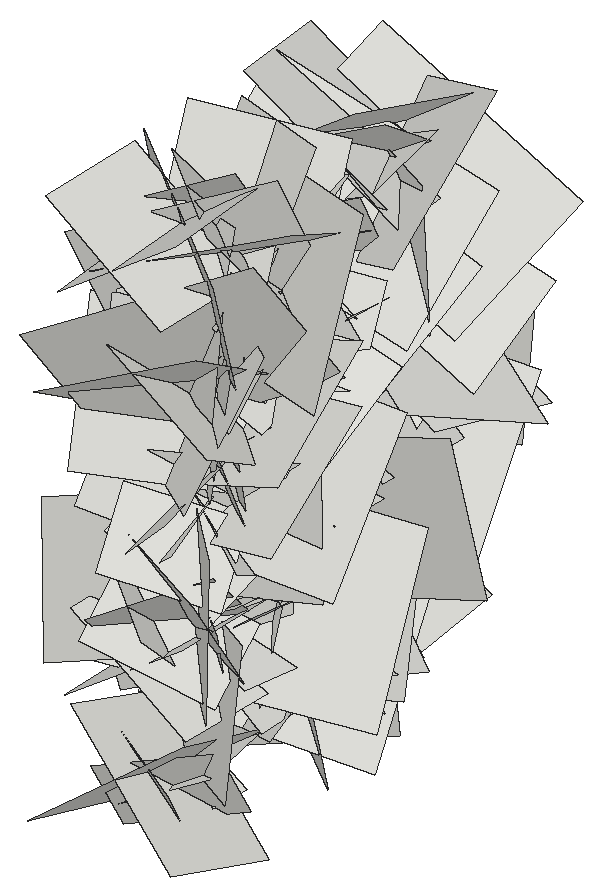
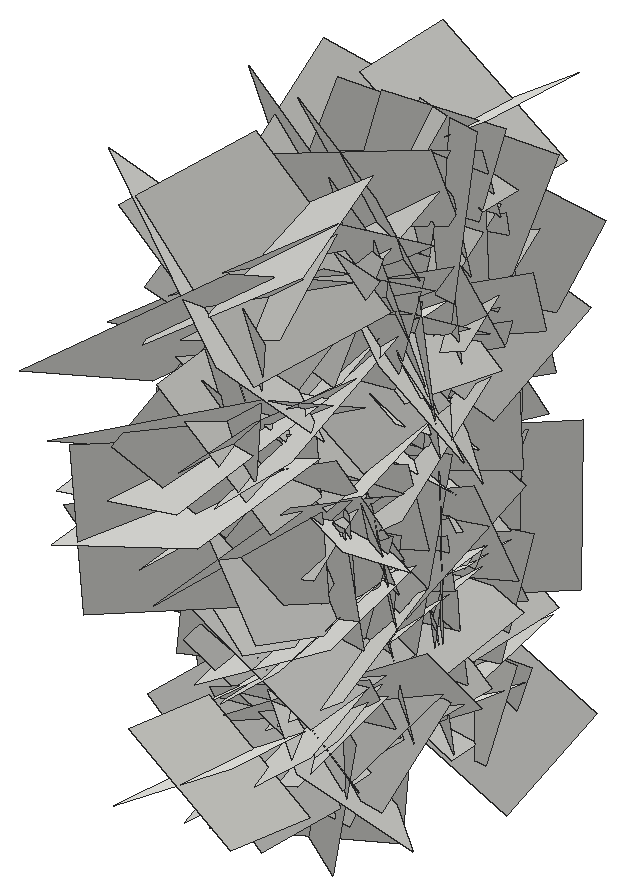
# SketchUp Ruby script. Lengths in inches.
U = 1.inch
M = Sketchup.active_model
def pt(a) = Geom::Point3d.new(a.map { |v| v * U })
def face(e, loops, mat)
  f = e.add_face(loops[0].map { |a| pt(a) })
  loops[1..].each { |l| e.add_face(l.map { |a| pt(a) }).erase! }
  f.material = f.back_material = mat if mat
  f
end
# faces: each face lists its corners as indices into pts; further lists are holes
def faces(e, pts, list, mat = nil) = list.each { |f| face(e, (f[0].is_a?(Array) ? f : [f]).map { |l| l.map { |i| pts[i] } }, mat) }
# xy, xz, yz: faces in a plane at the given z, y or x. An outline is a flat list of corners, or four numbers for a rectangle; further outlines are holes
def ring(l) = l.size == 4 ? [[l[0], l[1]], [l[2], l[1]], [l[2], l[3]], [l[0], l[3]]] : l.each_slice(2).to_a
def flat(e, list, mat, &to3) = list.each { |f| face(e, (f[0].is_a?(Array) ? f : [f]).map { |l| ring(l).map { |u, v| to3.(u, v) } }, mat) }
def xy(e, z, list, mat = nil) = flat(e, list, mat) { |x, y| [x, y, z] }
def xz(e, y, list, mat = nil) = flat(e, list, mat) { |x, z| [x, y, z] }
def yz(e, x, list, mat = nil) = flat(e, list, mat) { |y, z| [x, y, z] }
def lines(e, pts, list) = list.each { |a, b| e.add_line(pt(pts[a]), pt(pts[b])) }
# prism: a flat outline (further loops are holes) pulled along v
def prism(e, loops, v, mat = nil)
  f = face(e, loops, mat); d = Geom::Vector3d.new(v.map { |x| x * U })
  f.pushpull(f.normal.samedirection?(d) ? d.length : -d.length)
end
def box(e, o, s, mat = nil) = prism(e, [[o, [o[0] + s[0], o[1], o[2]], [o[0] + s[0], o[1] + s[1], o[2]], [o[0], o[1] + s[1], o[2]]]], [0, 0, s[2]], mat)
def at(x, y, z, deg = 0) = Geom::Transformation.translation(pt([x, y, z])) * Geom::Transformation.rotation(ORIGIN, Z_AXIS, deg.degrees)
def axes(o, x, y, z) = Geom::Transformation.new([*x, 0, *y, 0, *z, 0, *pt(o).to_a, 1])
def part(name) = M.definitions.add(name)
# library, detail: a bought-in or finely detailed component or shape, given as its bounding box
def library(name, o, s) = part(name).tap { |d| box(d.entities, o, s) }
def detail(e, o, s) = box(e.add_group.entities, o, s)
def put(e, d, t, mat = nil) = e.add_instance(d, t).tap { |i| i.material = mat if mat }
def group(e, t, mat = nil) = e.add_group.tap { |g| g.transformation = t; g.material = mat if mat }.entities
root = M.entities
c1 = part("Component\#6")
p = [[0.01,0,0],[0,3.24,4.54],[4.32,3.24,4.54],[4.33,0,0]]
faces(c1.entities,p,[[0,1,2,3]])
put(root,c1,axes([424.49,185.4,30.76],[0.02152,-0.00963,-1.2106],[0.23963,-1.18945,0.01326],[-1.26071,-0.22625,-0.01814]))
put(root,c1,axes([420.52,183.74,37.84],[0.08456,-0.37494,0.46177],[-0.03825,0.46199,0.38136],[0.62935,0.07846,-0.03886]))
put(root,c1,axes([420.52,188.62,32.29],[-0.0866,-0.74743,0.19758],[-0.06186,0.20408,0.74787],[0.81715,-0.06376,0.07755]))
put(root,c1,axes([420.52,184.65,28.76],[0.04824,-0.62434,-0.28052],[-0.09786,-0.28417,0.61748],[0.7189,0.00321,0.10288]))
put(root,c1,axes([424.49,186.48,30.64],[-0.03295,0.70699,0.47041],[-0.18441,0.45544,-0.69599],[-0.88105,-0.12176,0.12808]))
put(root,c1,axes([424.49,180.55,24.45],[-0.04702,0.95483,-0.28451],[0.08229,-0.28062,-0.95386],[-1.05288,-0.06457,-0.06184]))
put(root,c1,axes([424.49,184.8,33.37],[-0.19651,0.19461,-0.78555],[0.01158,-0.80522,-0.20206],[-0.85778,-0.05545,0.17724]))
put(root,c1,axes([424.49,181.12,36.49],[0.0887,0.85058,-0.45713],[-0.14057,-0.44437,-0.85112],[-1.01388,0.13603,0.07801]))
put(root,c1,axes([420.52,182.11,23.57],[-0.01533,0.32032,-0.55846],[0.07998,-0.55391,-0.31966],[0.67773,0.07262,0.02509]))
put(root,c1,axes([420.52,186.27,36.66],[-0.23271,0.08267,-1.0169],[-0.17131,-1.02986,-0.04883],[1.06781,-0.14721,-0.22945]))
put(root,c1,axes([420.52,181.88,29.24],[0.0732,0.47057,-0.46808],[-0.06498,-0.46407,-0.47558],[0.70054,-0.09222,0.00479]))
put(root,c1,axes([420.52,188.01,25.87],[-0.18323,0.88768,-0.1275],[-0.06793,-0.14175,-0.89995],[0.94816,0.16139,-0.08912]))
put(root,c1,axes([424.49,186.85,26],[-0.04759,0.74401,-0.43208],[-0.09551,-0.43435,-0.73856],[-0.90698,0.0067,0.10045]))
put(root,c1,axes([424.49,182.62,33.52],[0.16113,0.63843,0.91206],[0.00988,0.91976,-0.64538],[-1.18006,0.09488,0.11913]))
put(root,c1,axes([420.52,188.3,31.13],[-0.1103,-0.11339,-0.88165],[-0.13763,-0.87621,0.12802],[0.93214,-0.14279,-0.08543]))
put(root,c1,axes([424.49,182.86,27.86],[-0.00866,0.87216,-0.09866],[-0.12421,-0.09886,-0.86427],[-0.92206,0.00513,0.11735]))
put(root,c1,axes([420.52,188.48,31.6],[0.00806,0.51701,-0.38199],[0.06142,-0.38101,-0.51453],[0.67861,0.02834,0.0511]))
put(root,c1,axes([420.52,189.49,31],[-0.19159,0.03614,-0.77666],[0.1449,-0.78347,-0.06827],[0.81131,0.14846,-0.17121]))
put(root,c1,axes([424.49,186.8,27.07],[0.11611,-1.02809,0.5245],[0.14127,0.5346,1.02006],[-1.21522,-0.03608,0.16869]))
put(root,c1,axes([420.52,181.75,22.9],[0.07496,0.59984,0.04506],[0.05269,0.03939,-0.60235],[0.63545,-0.07402,0.04463]))
put(root,c1,axes([424.49,190.89,25.45],[0.07637,-0.93381,0.1535],[-0.06656,0.14888,0.93522],[-1.00091,-0.08115,-0.05048]))
put(root,c1,axes([424.49,189.24,21.76],[-0.15995,-0.688,0.38857],[0.02017,0.39231,0.70202],[-0.83731,0.14088,-0.05731]))
put(root,c1,axes([420.52,186.9,33.68],[-0.12726,-0.80704,-0.07778],[0.05104,-0.08559,0.81372],[0.85791,-0.11462,-0.05995]))
put(root,c1,axes([420.52,183.3,35.54],[0.06853,-0.0517,0.64839],[0.02911,0.65122,0.04919],[0.68886,-0.02238,-0.06659]))
put(root,c1,axes([424.49,182.91,34.72],[0.14912,-0.41506,0.98502],[0.044,0.99488,0.41329],[-1.13217,-0.016,0.1458]))
put(root,c1,axes([424.49,191.48,24.4],[0.24044,-0.84726,-0.84182],[0.11443,-0.83882,0.87332],[-1.26085,-0.2377,-0.08127]))
put(root,c1,axes([420.52,194.3125,23.26],[-0.02367,-0.75059,-0.08188],[0.02978,-0.08269,0.75031],[0.79979,-0.01914,-0.03036]))
put(root,c1,axes([424.49,189.58,22.99],[0.08755,-0.94666,0.34405],[0.04779,0.34833,0.94763],[-1.06661,-0.0621,0.0707]))
put(root,c1,axes([424.49,183.5625,38.07],[-0.03427,-0.86867,-0.02883],[0.01016,-0.0292,0.8692],[-0.92124,0.03199,0.01066]))
put(root,c1,axes([420.52,186.98,23.44],[-0.07046,0.41434,0.63319],[0.10971,0.63463,-0.40442],[0.79457,-0.05088,0.11199]))
put(root,c1,axes([424.49,186.99,20.26],[-0.04681,-0.17583,0.86867],[0.05724,0.86759,0.17835],[-0.93771,0.06173,-0.03248]))
put(root,c1,axes([420.52,182.78,23.92],[-0.06221,-0.24398,0.83625],[-0.07047,0.83695,0.23952],[0.92069,0.04758,0.07484]))
put(root,c1,axes([424.49,187.32,34.27],[-0.05201,-0.4187,0.7383],[0.02779,0.73844,0.42051],[-0.89926,0.04704,-0.0297]))
put(root,c1,axes([420.52,187.84,31.26],[0.01205,0.8882,0.30464],[-0.22592,0.29915,-0.86424],[0.96935,0.05868,-0.20521]))
put(root,c1,axes([420.52,187.61,26.86],[-0.07932,-0.16974,-0.83453],[-0.0041,-0.83766,0.17072],[0.9027,-0.01872,-0.07255]))
put(root,c1,axes([420.52,184.84,39.1],[0.02023,-0.20369,-0.6632],[0.11732,-0.65406,0.20407],[0.72599,0.11137,-0.0145]))
put(root,c1,axes([424.49,180.54,27.52],[-0.00647,0.86334,-0.00303],[0.00368,-0.003,-0.86336],[-0.91514,-0.00612,-0.00345]))
put(root,c1,axes([424.49,189.53,40.3125],[0.07096,0.70634,-0.4758],[-0.12627,-0.46481,-0.70678],[-0.89387,0.12173,0.06207]))
put(root,c1,axes([424.49,192.58,32.17],[-0.11188,-0.86522,-0.03173],[0.14554,-0.04829,0.85998],[-0.90613,0.09907,0.14204]))
put(root,c1,axes([424.49,185.86,28.71],[0.06844,0.29244,0.76285],[-0.17475,0.75415,-0.27515],[-0.84819,-0.13178,0.11824]))
put(root,c1,axes([420.52,188.23,41.22],[-0.26749,1.02168,-0.17372],[0.00845,-0.17688,-1.05183],[1.0985,0.25014,-0.03421]))
put(root,c1,axes([424.49,187.08,35.11],[0.23629,-0.52338,-1.02054],[0.13084,-1.02265,0.55142],[-1.20867,-0.21302,-0.13982]))
put(root,c1,axes([420.52,187.74,23.43],[-0.08523,-0.9506,0.05636],[-0.09187,0.06363,0.94959],[1.00521,-0.07479,0.09156]))
put(root,c1,axes([420.52,184.52,38.07],[-0.06477,0.36641,0.7198],[0.11209,0.71927,-0.35717],[0.84878,-0.06703,0.10209]))
put(root,c1,axes([420.52,184.92,37.05],[0.01613,-0.13323,-0.78421],[0.01491,-0.78419,0.1335],[0.84304,0.01642,0.01265]))
put(root,c1,axes([424.49,184.92,37.05],[-0.01613,-0.13323,-0.78421],[-0.01491,-0.78419,0.1335],[-0.84304,0.01642,0.01265]))
put(root,c1,axes([424.49,184.52,38.07],[0.06477,0.36641,0.7198],[-0.11209,0.71927,-0.35717],[-0.84878,-0.06703,0.10209]))
put(root,c1,axes([424.49,187.74,23.43],[0.08523,-0.9506,0.05636],[0.09187,0.06363,0.94959],[-1.00521,-0.07479,0.09156]))
put(root,c1,axes([420.52,187.08,35.11],[-0.23629,-0.52338,-1.02054],[-0.13084,-1.02265,0.55142],[1.20867,-0.21302,-0.13982]))
put(root,c1,axes([424.49,188.23,41.22],[0.26749,1.02168,-0.17372],[-0.00845,-0.17688,-1.05183],[-1.0985,0.25014,-0.03421]))
put(root,c1,axes([420.52,185.86,28.71],[-0.06844,0.29244,0.76285],[0.17475,0.75415,-0.27515],[0.84819,-0.13178,0.11824]))
put(root,c1,axes([420.52,192.58,32.17],[0.11188,-0.86522,-0.03173],[-0.14554,-0.04829,0.85998],[0.90613,0.09907,0.14204]))
put(root,c1,axes([420.52,189.53,40.3125],[-0.07096,0.70634,-0.4758],[0.12627,-0.46481,-0.70678],[0.89387,0.12173,0.06207]))
put(root,c1,axes([420.52,180.54,27.52],[0.00647,0.86334,-0.00303],[-0.00368,-0.003,-0.86336],[0.91514,-0.00612,-0.00345]))
put(root,c1,axes([424.49,184.84,39.1],[-0.02023,-0.20369,-0.6632],[-0.11732,-0.65406,0.20407],[-0.72599,0.11137,-0.0145]))
put(root,c1,axes([424.49,187.61,26.86],[0.07932,-0.16974,-0.83453],[0.0041,-0.83766,0.17072],[-0.9027,-0.01872,-0.07255]))
put(root,c1,axes([424.49,187.84,31.26],[-0.01205,0.8882,0.30464],[0.22592,0.29915,-0.86424],[-0.96935,0.05868,-0.20521]))
put(root,c1,axes([420.52,187.32,34.27],[0.05201,-0.4187,0.7383],[-0.02779,0.73844,0.42051],[0.89926,0.04704,-0.0297]))
put(root,c1,axes([424.49,182.78,23.92],[0.06221,-0.24398,0.83625],[0.07047,0.83695,0.23952],[-0.92069,0.04758,0.07484]))
put(root,c1,axes([420.52,186.99,20.26],[0.04681,-0.17583,0.86867],[-0.05724,0.86759,0.17835],[0.93771,0.06173,-0.03248]))
put(root,c1,axes([424.49,186.98,23.44],[0.07046,0.41434,0.63319],[-0.10971,0.63463,-0.40442],[-0.79457,-0.05088,0.11199]))
put(root,c1,axes([420.52,183.5625,38.07],[0.03427,-0.86867,-0.02883],[-0.01016,-0.0292,0.8692],[0.92124,0.03199,0.01066]))
put(root,c1,axes([420.52,189.58,22.99],[-0.08755,-0.94666,0.34405],[-0.04779,0.34833,0.94763],[1.06661,-0.0621,0.0707]))
put(root,c1,axes([424.49,194.3125,23.26],[0.02367,-0.75059,-0.08188],[-0.02978,-0.08269,0.75031],[-0.79979,-0.01914,-0.03036]))
put(root,c1,axes([420.52,191.48,24.4],[-0.24044,-0.84726,-0.84182],[-0.11443,-0.83882,0.87332],[1.26085,-0.2377,-0.08127]))
put(root,c1,axes([420.52,182.91,34.72],[-0.14912,-0.41506,0.98502],[-0.044,0.99488,0.41329],[1.13217,-0.016,0.1458]))
put(root,c1,axes([424.49,183.3,35.54],[-0.06853,-0.0517,0.64839],[-0.02911,0.65122,0.04919],[-0.68886,-0.02238,-0.06659]))
put(root,c1,axes([424.49,186.9,33.68],[0.12726,-0.80704,-0.07778],[-0.05104,-0.08559,0.81372],[-0.85791,-0.11462,-0.05995]))
put(root,c1,axes([420.52,189.24,21.76],[0.15995,-0.688,0.38857],[-0.02017,0.39231,0.70202],[0.83731,0.14088,-0.05731]))
put(root,c1,axes([420.52,190.89,25.45],[-0.07637,-0.93381,0.1535],[0.06656,0.14888,0.93522],[1.00091,-0.08115,-0.05048]))
put(root,c1,axes([424.49,181.75,22.9],[-0.07496,0.59984,0.04506],[-0.05269,0.03939,-0.60235],[-0.63545,-0.07402,0.04463]))
put(root,c1,axes([420.52,186.8,27.07],[-0.11611,-1.02809,0.5245],[-0.14127,0.5346,1.02006],[1.21522,-0.03608,0.16869]))
put(root,c1,axes([424.49,189.49,31],[0.19159,0.03614,-0.77666],[-0.1449,-0.78347,-0.06827],[-0.81131,0.14846,-0.17121]))
put(root,c1,axes([424.49,188.48,31.6],[-0.00806,0.51701,-0.38199],[-0.06142,-0.38101,-0.51453],[-0.67861,0.02834,0.0511]))
put(root,c1,axes([420.52,182.86,27.86],[0.00866,0.87216,-0.09866],[0.12421,-0.09886,-0.86427],[0.92206,0.00513,0.11735]))
put(root,c1,axes([424.49,188.3,31.13],[0.1103,-0.11339,-0.88165],[0.13763,-0.87621,0.12802],[-0.93214,-0.14279,-0.08543]))
put(root,c1,axes([420.52,182.62,33.52],[-0.16113,0.63843,0.91206],[-0.00988,0.91976,-0.64538],[1.18006,0.09488,0.11913]))
put(root,c1,axes([420.52,186.85,26],[0.04759,0.74401,-0.43208],[0.09551,-0.43435,-0.73856],[0.90698,0.0067,0.10045]))
put(root,c1,axes([424.49,188.01,25.87],[0.18323,0.88768,-0.1275],[0.06793,-0.14175,-0.89995],[-0.94816,0.16139,-0.08912]))
put(root,c1,axes([424.49,181.88,29.24],[-0.0732,0.47057,-0.46808],[0.06498,-0.46407,-0.47558],[-0.70054,-0.09222,0.00479]))
put(root,c1,axes([424.49,186.27,36.66],[0.23271,0.08267,-1.0169],[0.17131,-1.02986,-0.04883],[-1.06781,-0.14721,-0.22945]))
put(root,c1,axes([424.49,182.11,23.57],[0.01533,0.32032,-0.55846],[-0.07998,-0.55391,-0.31966],[-0.67773,0.07262,0.02509]))
put(root,c1,axes([420.52,181.12,36.49],[-0.0887,0.85058,-0.45713],[0.14057,-0.44437,-0.85112],[1.01388,0.13603,0.07801]))
put(root,c1,axes([420.52,184.8,33.37],[0.19651,0.19461,-0.78555],[-0.01158,-0.80522,-0.20206],[0.85778,-0.05545,0.17724]))
put(root,c1,axes([420.52,180.55,24.45],[0.04702,0.95483,-0.28451],[-0.08229,-0.28062,-0.95386],[1.05288,-0.06457,-0.06184]))
put(root,c1,axes([420.52,186.48,30.64],[0.03295,0.70699,0.47041],[0.18441,0.45544,-0.69599],[0.88105,-0.12176,0.12808]))
put(root,c1,axes([424.49,184.65,28.76],[-0.04824,-0.62434,-0.28052],[0.09786,-0.28417,0.61748],[-0.7189,0.00321,0.10288]))
put(root,c1,axes([424.49,188.62,32.29],[0.0866,-0.74743,0.19758],[0.06186,0.20408,0.74787],[-0.81715,-0.06376,0.07755]))
put(root,c1,axes([424.49,183.74,37.84],[-0.08456,-0.37494,0.46177],[0.03825,0.46199,0.38136],[-0.62935,0.07846,-0.03886]))
put(root,c1,axes([420.52,185.4,30.76],[-0.02152,-0.00963,-1.2106],[-0.23963,-1.18945,0.01326],[1.26071,-0.22625,-0.01814]))
put(root,c1,axes([420.52,187.18,35.87],[-0.21905,1.32848,-0.23139],[-0.18572,-0.25856,-1.32798],[1.41727,0.17144,-0.20979]))
put(root,c1,axes([424.49,188.41,35.3125],[-0.03073,0.48255,0.4704],[0.10717,0.46862,-0.47449],[-0.70624,0.05011,-0.09248]))
put(root,c1,axes([424.49,183.98,26.9],[0.15473,-0.64925,-0.29626],[-0.07231,-0.3137,0.65387],[-0.75301,-0.10329,-0.12366]))
put(root,c1,axes([424.49,183.4375,30.23],[0.10865,-0.24445,0.66529],[-0.00738,0.67183,0.24793],[-0.75127,-0.04195,0.09378]))
put(root,c1,axes([424.49,185.35,37.93],[0.06077,0.5182,0.40006],[-0.00909,0.40215,-0.51968],[-0.69387,0.04012,0.04185]))
put(root,c1,axes([420.52,182.41,31.86],[-0.21699,-0.67676,1.03332],[0.0082,1.04669,0.68705],[1.3093,-0.11872,0.16695]))
put(root,c1,axes([420.52,181.64,30.57],[0.02444,0.48831,-0.77146],[0.19424,-0.75848,-0.47462],[0.9481,0.1428,0.11713]))
put(root,c1,axes([420.52,184.85,32.98],[-0.15473,1.07562,-0.16592],[0.16403,-0.14519,-1.07739],[1.14193,0.1666,0.13228]))
put(root,c1,axes([424.49,179.78,31.84],[0.01485,0.68647,0.23212],[0.1576,0.2245,-0.67291],[-0.75179,0.06062,-0.13648]))
put(root,c1,axes([424.49,188.93,38.32],[0.06934,0.59373,0.25],[-0.00198,0.25145,-0.59671],[-0.68287,0.05956,0.02711]))
put(root,c1,axes([424.49,193.29,29.97],[-0.02765,-0.60791,0.13872],[0.08921,0.13414,0.60366],[-0.6549,0.04394,0.07638]))
put(root,c1,axes([420.52,189.07,22.99],[0.09993,-0.91741,-0.05408],[0.10319,-0.04408,0.91762],[0.96866,0.09934,-0.09218]))
put(root,c1,axes([420.52,185.63,37.94],[-0.10296,1.07287,0.66666],[-0.13207,0.65722,-1.07584],[1.33238,0.14805,-0.05512]))
put(root,c1,axes([420.52,185.55,26.35],[0.05433,-0.24183,-1.04679],[-0.06418,-1.04696,0.23891],[1.13701,-0.04754,0.0635]))
put(root,c1,axes([424.49,186.02,29.02],[0.12909,0.32312,-0.64935],[0.06195,-0.66067,-0.31779],[-0.76632,0.00102,-0.13508]))
put(root,c1,axes([420.52,190.19,31.82],[0.07854,-1.04848,0.11995],[-0.05802,0.11627,1.05008],[1.11713,0.07975,0.0461]))
put(root,c1,axes([424.49,188.83,29.07],[0.04972,0.59189,0.16701],[0.02122,0.16593,-0.59371],[-0.65156,0.05057,-0.00659]))
put(root,c1,axes([420.52,185.29,39.56],[0.11827,0.82487,-0.51088],[0.03346,-0.51706,-0.82795],[1.02793,-0.07808,0.08573]))
put(root,c1,axes([420.52,186.92,28.87],[0.11772,1.08189,-0.3436],[-0.18933,-0.32428,-1.0788],[1.18826,-0.15885,-0.13785]))
put(root,c1,axes([424.49,191.45,35.51],[0.13227,0.51495,-0.41011],[0.00116,-0.41758,-0.52399],[-0.6978,0.09692,-0.07861]))
put(root,c1,axes([424.49,183.51,30.36],[0.10644,-0.42009,-0.4575],[-0.01901,-0.46521,0.42323],[-0.65811,-0.0545,-0.08622]))
put(root,c1,axes([420.52,184.16,23.6],[0.00632,0.19994,1.20323],[-0.15077,1.19515,-0.1979],[1.28409,0.13934,-0.02916]))
put(root,c1,axes([420.52,189.26,31.29],[0.07003,-0.18149,-1.00879],[0.05402,-1.00905,0.18487],[1.08514,0.06195,0.0559]))
put(root,c1,axes([424.49,191.07,24.72],[0.08022,-0.60182,-0.03468],[0.03515,-0.03074,0.60586],[-0.63802,-0.07736,0.02902]))
put(root,c1,axes([420.52,187.65,25.55],[0.14301,-0.32766,0.90945],[0.11586,0.91755,0.31436],[1.01811,-0.05839,-0.16352]))
put(root,c1,axes([420.52,192.86,38.11],[0.10772,-0.0541,-1.0459],[0.04447,-1.04976,0.05837],[1.10925,0.04734,0.09923]))
put(root,c1,axes([424.49,188.74,27.6],[0.13014,-0.45431,-0.37588],[0.00674,-0.3829,0.46487],[-0.62498,-0.09873,-0.07326]))
put(root,c1,axes([420.52,181.98,27.65],[0.03848,-0.07343,1.06513],[0.13392,1.05855,0.06867],[1.12376,-0.12364,-0.04466]))
put(root,c1,axes([420.52,182.88,33.98],[0.05541,0.90127,0.55592],[0.17138,0.54328,-0.89597],[1.1093,-0.12895,0.11065]))
put(root,c1,axes([420.52,190.1,29],[0.15352,-0.05709,1.12322],[-0.06907,1.13017,0.06585],[1.19015,0.07295,-0.14107]))
put(root,c1,axes([420.52,185.59,36.56],[0.07365,1.00309,0.56692],[0.00038,0.56794,-1.00493],[1.22135,-0.06067,-0.03387]))
put(root,c1,axes([420.52,194.96,38.36],[-0.08597,-0.96025,-0.92678],[-0.03419,-0.92681,0.9631],[1.41421,-0.08078,-0.03305]))
put(root,c1,axes([420.52,188.57,34.3],[-0.02784,1.05016,0.5271],[0.1514,0.52617,-1.0412],[1.23628,-0.04079,0.13938]))
put(root,c1,axes([420.52,186.91,28.91],[-0.08475,0.77289,1.06783],[0.0494,1.07079,-0.77154],[1.39641,0.00903,0.0921]))
put(root,c1,axes([420.52,187.29,32.09],[-0.03087,-0.89426,-0.74249],[0.26998,-0.72958,0.86873],[1.20212,0.14089,-0.21417]))
put(root,c1,axes([420.52,190.5,33.59],[0.11278,1.05886,-0.21225],[0.21462,-0.22906,-1.04119],[1.12442,-0.06248,0.22002]))
put(root,c1,axes([420.52,184.99,36.41],[0.13687,-0.99381,0.45239],[0.15227,0.46704,0.985],[1.14738,0.05657,-0.18469]))
put(root,c1,axes([420.52,181.61,25.33],[-0.14764,0.72138,1.18272],[0.09804,1.19088,-0.71546],[1.46521,-0.007,0.16705]))
put(root,c1,axes([420.52,187.26,33.24],[0.066,-0.95024,-0.64083],[0.19237,-0.6255,0.94515],[1.19957,0.15259,-0.11631]))
put(root,c1,axes([420.52,188.72,38.18],[0.108,1.17484,0.54266],[-0.09899,0.5496,-1.17232],[1.36819,-0.05298,-0.12766]))
put(root,c1,axes([420.52,180.73,30.67],[0.05707,0.69485,1.12415],[-0.04583,1.1254,-0.69356],[1.4001,0.00851,-0.06852]))
put(root,c1,axes([420.52,188.1875,39.24],[0.00053,-0.50504,-1.25708],[0.1621,-1.24903,0.50186],[1.42684,0.14209,-0.05655]))
put(root,c1,axes([420.52,186.51,25.44],[-0.00901,-0.3677,1.34811],[0.26845,1.32541,0.3631],[1.45667,-0.24653,-0.05858]))
put(root,c1,axes([420.52,190.14,35.27],[0.30668,1.10496,-0.445],[0.14325,-0.48543,-1.11748],[1.25452,-0.21469,0.23639]))
